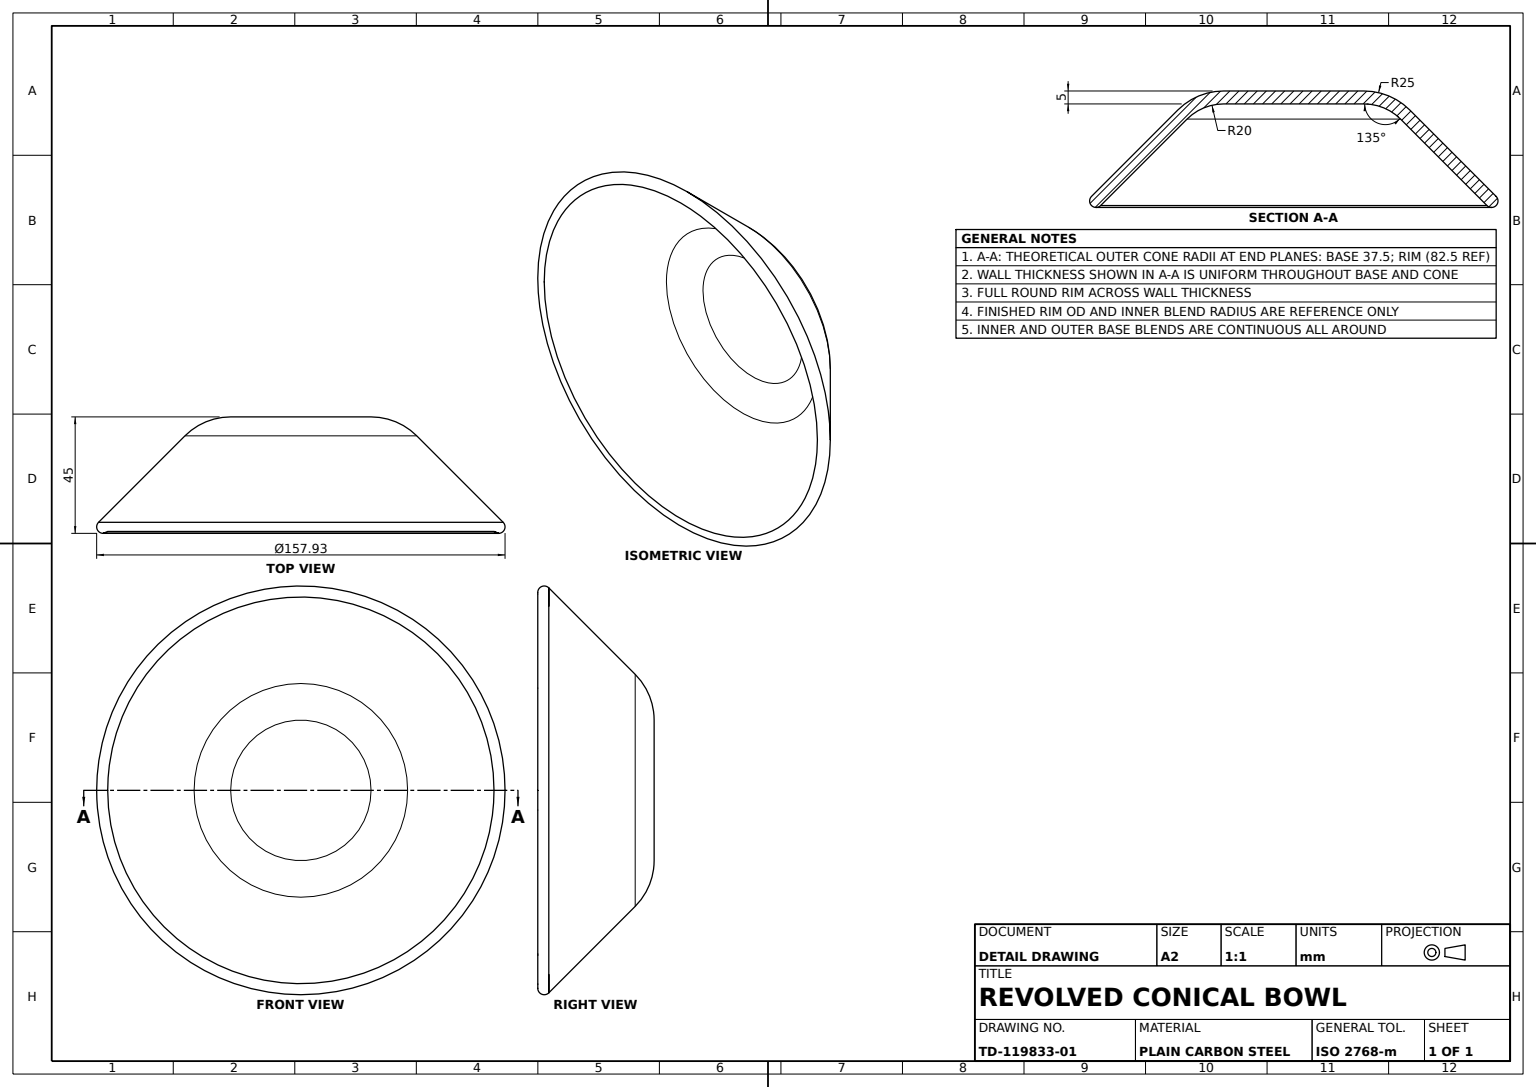
ISO-10303-21;
HEADER;
FILE_DESCRIPTION((''),'2;1');
FILE_NAME('','',(''),(''),'','','');
FILE_SCHEMA(('AUTOMOTIVE_DESIGN'));
ENDSEC;
DATA;
#1=APPLICATION_CONTEXT('');
#2=PRODUCT_CONTEXT('',#1,'mechanical');
#3=PRODUCT('','','',(#2));
#4=PRODUCT_DEFINITION_FORMATION('','',#3);
#5=PRODUCT_DEFINITION_CONTEXT('',#1,'design');
#6=PRODUCT_DEFINITION('','',#4,#5);
#7=PRODUCT_DEFINITION_SHAPE('','',#6);
#8=(LENGTH_UNIT()NAMED_UNIT(*)SI_UNIT(.MILLI.,.METRE.));
#9=(NAMED_UNIT(*)PLANE_ANGLE_UNIT()SI_UNIT($,.RADIAN.));
#10=(NAMED_UNIT(*)SI_UNIT($,.STERADIAN.)SOLID_ANGLE_UNIT());
#11=UNCERTAINTY_MEASURE_WITH_UNIT(LENGTH_MEASURE(1.E-05),#8,'distance_accuracy_value','');
#12=(GEOMETRIC_REPRESENTATION_CONTEXT(3)GLOBAL_UNCERTAINTY_ASSIGNED_CONTEXT((#11))GLOBAL_UNIT_ASSIGNED_CONTEXT((#8,#9,#10))REPRESENTATION_CONTEXT('',''));
#13=CARTESIAN_POINT('',(0.,40.732233,-78.232233));
#14=VERTEX_POINT('',#13);
#15=CARTESIAN_POINT('',(0.,44.267767,-74.696699));
#16=VERTEX_POINT('',#15);
#17=CARTESIAN_POINT('',(0.,41.910744,-79.410744));
#18=CARTESIAN_POINT('',(0.,44.267767,-80.));
#19=CARTESIAN_POINT('',(0.,46.035534,-78.232233));
#20=CARTESIAN_POINT('',(0.,45.446278,-75.87521));
#21=(BOUNDED_CURVE()B_SPLINE_CURVE(5,(#13,#17,#18,#19,#20,#15),.UNSPECIFIED.,.F.,.T.)B_SPLINE_CURVE_WITH_KNOTS((6,6),(0.,1.),.UNSPECIFIED.)CURVE()GEOMETRIC_REPRESENTATION_ITEM()RATIONAL_B_SPLINE_CURVE((1.,0.6,0.4,0.4,0.6,1.))REPRESENTATION_ITEM(''));
#22=EDGE_CURVE('',#14,#16,#21,.T.);
#23=ORIENTED_EDGE('',*,*,#22,.T.);
#24=CARTESIAN_POINT('',(0.,44.267767,74.696699));
#25=VERTEX_POINT('',#24);
#26=CARTESIAN_POINT('',(4.888888,44.267767,74.696699));
#27=CARTESIAN_POINT('',(9.777654,44.267767,74.215198));
#28=CARTESIAN_POINT('',(19.367552,44.267767,72.307648));
#29=CARTESIAN_POINT('',(24.068446,44.267767,70.881648));
#30=CARTESIAN_POINT('',(33.101932,44.267767,67.139855));
#31=CARTESIAN_POINT('',(37.434301,44.267767,64.824156));
#32=CARTESIAN_POINT('',(45.564224,44.267767,59.391915));
#33=CARTESIAN_POINT('',(49.361577,44.267767,56.275508));
#34=CARTESIAN_POINT('',(56.275508,44.267767,49.361577));
#35=CARTESIAN_POINT('',(59.391915,44.267767,45.564224));
#36=CARTESIAN_POINT('',(64.824156,44.267767,37.434301));
#37=CARTESIAN_POINT('',(67.139855,44.267767,33.101932));
#38=CARTESIAN_POINT('',(70.881648,44.267767,24.068446));
#39=CARTESIAN_POINT('',(72.307648,44.267767,19.367552));
#40=CARTESIAN_POINT('',(74.215198,44.267767,9.777654));
#41=CARTESIAN_POINT('',(74.696699,44.267767,4.888888));
#42=CARTESIAN_POINT('',(74.696699,44.267767,-4.888888));
#43=CARTESIAN_POINT('',(74.215198,44.267767,-9.777654));
#44=CARTESIAN_POINT('',(72.307648,44.267767,-19.367552));
#45=CARTESIAN_POINT('',(70.881648,44.267767,-24.068446));
#46=CARTESIAN_POINT('',(67.139855,44.267767,-33.101932));
#47=CARTESIAN_POINT('',(64.824156,44.267767,-37.434301));
#48=CARTESIAN_POINT('',(59.391915,44.267767,-45.564224));
#49=CARTESIAN_POINT('',(56.275508,44.267767,-49.361577));
#50=CARTESIAN_POINT('',(49.361577,44.267767,-56.275508));
#51=CARTESIAN_POINT('',(45.564224,44.267767,-59.391915));
#52=CARTESIAN_POINT('',(37.434301,44.267767,-64.824156));
#53=CARTESIAN_POINT('',(33.101932,44.267767,-67.139855));
#54=CARTESIAN_POINT('',(24.068446,44.267767,-70.881648));
#55=CARTESIAN_POINT('',(19.367552,44.267767,-72.307648));
#56=CARTESIAN_POINT('',(9.777654,44.267767,-74.215198));
#57=CARTESIAN_POINT('',(4.888888,44.267767,-74.696699));
#58=B_SPLINE_CURVE_WITH_KNOTS('',3,(#24,#26,#27,#28,#29,#30,#31,#32,#33,#34,#35,#36,#37,#38,#39,#40,#41,#42,#43,#44,#45,#46,#47,#48,#49,#50,#51,#52,#53,#54,#55,#56,#57,#15),.UNSPECIFIED.,.F.,.F.,(4,2,2,2,2,2,2,2,2,2,2,2,2,2,2,2,4),(0.,0.03125,0.0625,0.09375,0.125,0.15625,0.1875,0.21875,0.25,0.28125,0.3125,0.34375,0.375,0.40625,0.4375,0.46875,0.5),.UNSPECIFIED.);
#59=EDGE_CURVE('',#25,#16,#58,.T.);
#60=ORIENTED_EDGE('',*,*,#59,.F.);
#61=CARTESIAN_POINT('',(0.,40.732233,78.232233));
#62=VERTEX_POINT('',#61);
#63=CARTESIAN_POINT('',(0.,41.910744,79.410744));
#64=CARTESIAN_POINT('',(0.,44.267767,80.));
#65=CARTESIAN_POINT('',(0.,46.035534,78.232233));
#66=CARTESIAN_POINT('',(0.,45.446278,75.87521));
#67=(BOUNDED_CURVE()B_SPLINE_CURVE(5,(#61,#63,#64,#65,#66,#24),.UNSPECIFIED.,.F.,.T.)B_SPLINE_CURVE_WITH_KNOTS((6,6),(0.,1.),.UNSPECIFIED.)CURVE()GEOMETRIC_REPRESENTATION_ITEM()RATIONAL_B_SPLINE_CURVE((1.,0.6,0.4,0.4,0.6,1.))REPRESENTATION_ITEM(''));
#68=EDGE_CURVE('',#62,#25,#67,.T.);
#69=ORIENTED_EDGE('',*,*,#68,.F.);
#70=CARTESIAN_POINT('',(5.120288,40.732233,-78.232233));
#71=CARTESIAN_POINT('',(10.240449,40.732233,-77.727941));
#72=CARTESIAN_POINT('',(20.284254,40.732233,-75.730104));
#73=CARTESIAN_POINT('',(25.20765,40.732233,-74.236608));
#74=CARTESIAN_POINT('',(34.668708,40.732233,-70.31771));
#75=CARTESIAN_POINT('',(39.206136,40.732233,-67.892404));
#76=CARTESIAN_POINT('',(47.720864,40.732233,-62.203045));
#77=CARTESIAN_POINT('',(51.697952,40.732233,-58.939133));
#78=CARTESIAN_POINT('',(58.939133,40.732233,-51.697952));
#79=CARTESIAN_POINT('',(62.203045,40.732233,-47.720864));
#80=CARTESIAN_POINT('',(67.892404,40.732233,-39.206136));
#81=CARTESIAN_POINT('',(70.31771,40.732233,-34.668708));
#82=CARTESIAN_POINT('',(74.236608,40.732233,-25.20765));
#83=CARTESIAN_POINT('',(75.730104,40.732233,-20.284254));
#84=CARTESIAN_POINT('',(77.727941,40.732233,-10.240449));
#85=CARTESIAN_POINT('',(78.232233,40.732233,-5.120288));
#86=CARTESIAN_POINT('',(78.232233,40.732233,5.120288));
#87=CARTESIAN_POINT('',(77.727941,40.732233,10.240449));
#88=CARTESIAN_POINT('',(75.730104,40.732233,20.284254));
#89=CARTESIAN_POINT('',(74.236608,40.732233,25.20765));
#90=CARTESIAN_POINT('',(70.31771,40.732233,34.668708));
#91=CARTESIAN_POINT('',(67.892404,40.732233,39.206136));
#92=CARTESIAN_POINT('',(62.203045,40.732233,47.720864));
#93=CARTESIAN_POINT('',(58.939133,40.732233,51.697952));
#94=CARTESIAN_POINT('',(51.697952,40.732233,58.939133));
#95=CARTESIAN_POINT('',(47.720864,40.732233,62.203045));
#96=CARTESIAN_POINT('',(39.206136,40.732233,67.892404));
#97=CARTESIAN_POINT('',(34.668708,40.732233,70.31771));
#98=CARTESIAN_POINT('',(25.20765,40.732233,74.236608));
#99=CARTESIAN_POINT('',(20.284254,40.732233,75.730104));
#100=CARTESIAN_POINT('',(10.240449,40.732233,77.727941));
#101=CARTESIAN_POINT('',(5.120288,40.732233,78.232233));
#102=B_SPLINE_CURVE_WITH_KNOTS('',3,(#13,#70,#71,#72,#73,#74,#75,#76,#77,#78,#79,#80,#81,#82,#83,#84,#85,#86,#87,#88,#89,#90,#91,#92,#93,#94,#95,#96,#97,#98,#99,#100,#101,#61),.UNSPECIFIED.,.F.,.F.,(4,2,2,2,2,2,2,2,2,2,2,2,2,2,2,2,4),(0.5,0.53125,0.5625,0.59375,0.625,0.65625,0.6875,0.71875,0.75,0.78125,0.8125,0.84375,0.875,0.90625,0.9375,0.96875,1.),.UNSPECIFIED.);
#103=EDGE_CURVE('',#14,#62,#102,.T.);
#104=ORIENTED_EDGE('',*,*,#103,.F.);
#105=EDGE_LOOP('',(#23,#60,#69,#104));
#106=FACE_OUTER_BOUND('',#105,.T.);
#107=CARTESIAN_POINT('',(-5.116753,40.732233,78.232233));
#108=CARTESIAN_POINT('',(-10.238436,40.732233,77.728342));
#109=CARTESIAN_POINT('',(-20.286267,40.732233,75.729704));
#110=CARTESIAN_POINT('',(-25.210916,40.732233,74.235256));
#111=CARTESIAN_POINT('',(-34.665443,40.732233,70.319062));
#112=CARTESIAN_POINT('',(-39.20443,40.732233,67.893544));
#113=CARTESIAN_POINT('',(-47.72257,40.732233,62.201905));
#114=CARTESIAN_POINT('',(-51.700451,40.732233,58.936634));
#115=CARTESIAN_POINT('',(-58.936634,40.732233,51.700451));
#116=CARTESIAN_POINT('',(-62.201905,40.732233,47.72257));
#117=CARTESIAN_POINT('',(-67.893544,40.732233,39.20443));
#118=CARTESIAN_POINT('',(-70.319062,40.732233,34.665443));
#119=CARTESIAN_POINT('',(-74.235256,40.732233,25.210916));
#120=CARTESIAN_POINT('',(-75.729704,40.732233,20.286267));
#121=CARTESIAN_POINT('',(-77.728342,40.732233,10.238436));
#122=CARTESIAN_POINT('',(-78.232233,40.732233,5.116753));
#123=CARTESIAN_POINT('',(-78.232233,40.732233,-5.116753));
#124=CARTESIAN_POINT('',(-77.728342,40.732233,-10.238436));
#125=CARTESIAN_POINT('',(-75.729704,40.732233,-20.286267));
#126=CARTESIAN_POINT('',(-74.235256,40.732233,-25.210916));
#127=CARTESIAN_POINT('',(-70.319062,40.732233,-34.665443));
#128=CARTESIAN_POINT('',(-67.893544,40.732233,-39.20443));
#129=CARTESIAN_POINT('',(-62.201905,40.732233,-47.72257));
#130=CARTESIAN_POINT('',(-58.936634,40.732233,-51.700451));
#131=CARTESIAN_POINT('',(-51.700451,40.732233,-58.936634));
#132=CARTESIAN_POINT('',(-47.72257,40.732233,-62.201905));
#133=CARTESIAN_POINT('',(-39.20443,40.732233,-67.893544));
#134=CARTESIAN_POINT('',(-34.665443,40.732233,-70.319062));
#135=CARTESIAN_POINT('',(-25.210916,40.732233,-74.235256));
#136=CARTESIAN_POINT('',(-20.286267,40.732233,-75.729704));
#137=CARTESIAN_POINT('',(-10.238436,40.732233,-77.728342));
#138=CARTESIAN_POINT('',(-5.116753,40.732233,-78.232233));
#139=CARTESIAN_POINT('',(5.116753,40.732233,-78.232233));
#140=CARTESIAN_POINT('',(10.238436,40.732233,-77.728342));
#141=CARTESIAN_POINT('',(20.286267,40.732233,-75.729704));
#142=CARTESIAN_POINT('',(25.210916,40.732233,-74.235256));
#143=CARTESIAN_POINT('',(34.665443,40.732233,-70.319062));
#144=CARTESIAN_POINT('',(39.20443,40.732233,-67.893544));
#145=CARTESIAN_POINT('',(47.72257,40.732233,-62.201905));
#146=CARTESIAN_POINT('',(51.700451,40.732233,-58.936634));
#147=CARTESIAN_POINT('',(58.936634,40.732233,-51.700451));
#148=CARTESIAN_POINT('',(62.201905,40.732233,-47.72257));
#149=CARTESIAN_POINT('',(67.893544,40.732233,-39.20443));
#150=CARTESIAN_POINT('',(70.319062,40.732233,-34.665443));
#151=CARTESIAN_POINT('',(74.235256,40.732233,-25.210916));
#152=CARTESIAN_POINT('',(75.729704,40.732233,-20.286267));
#153=CARTESIAN_POINT('',(77.728342,40.732233,-10.238436));
#154=CARTESIAN_POINT('',(78.232233,40.732233,-5.116753));
#155=CARTESIAN_POINT('',(78.232233,40.732233,5.116753));
#156=CARTESIAN_POINT('',(77.728342,40.732233,10.238436));
#157=CARTESIAN_POINT('',(75.729704,40.732233,20.286267));
#158=CARTESIAN_POINT('',(74.235256,40.732233,25.210916));
#159=CARTESIAN_POINT('',(70.319062,40.732233,34.665443));
#160=CARTESIAN_POINT('',(67.893544,40.732233,39.20443));
#161=CARTESIAN_POINT('',(62.201905,40.732233,47.72257));
#162=CARTESIAN_POINT('',(58.936634,40.732233,51.700451));
#163=CARTESIAN_POINT('',(51.700451,40.732233,58.936634));
#164=CARTESIAN_POINT('',(47.72257,40.732233,62.201905));
#165=CARTESIAN_POINT('',(39.20443,40.732233,67.893544));
#166=CARTESIAN_POINT('',(34.665443,40.732233,70.319062));
#167=CARTESIAN_POINT('',(25.210916,40.732233,74.235256));
#168=CARTESIAN_POINT('',(20.286267,40.732233,75.729704));
#169=CARTESIAN_POINT('',(10.238436,40.732233,77.728342));
#170=CARTESIAN_POINT('',(5.116753,40.732233,78.232233));
#171=CARTESIAN_POINT('',(-5.194863,41.910744,79.410744));
#172=CARTESIAN_POINT('',(-10.393185,41.910744,78.89916));
#173=CARTESIAN_POINT('',(-20.591351,41.910744,76.870618));
#174=CARTESIAN_POINT('',(-25.589749,41.910744,75.353949));
#175=CARTESIAN_POINT('',(-35.188604,41.910744,71.377973));
#176=CARTESIAN_POINT('',(-39.795452,41.910744,68.916019));
#177=CARTESIAN_POINT('',(-48.44104,41.910744,63.139222));
#178=CARTESIAN_POINT('',(-52.478553,41.910744,59.825199));
#179=CARTESIAN_POINT('',(-59.825199,41.910744,52.478553));
#180=CARTESIAN_POINT('',(-63.139222,41.910744,48.44104));
#181=CARTESIAN_POINT('',(-68.916019,41.910744,39.795452));
#182=CARTESIAN_POINT('',(-71.377973,41.910744,35.188604));
#183=CARTESIAN_POINT('',(-75.353949,41.910744,25.589749));
#184=CARTESIAN_POINT('',(-76.870618,41.910744,20.591351));
#185=CARTESIAN_POINT('',(-78.89916,41.910744,10.393185));
#186=CARTESIAN_POINT('',(-79.410744,41.910744,5.194863));
#187=CARTESIAN_POINT('',(-79.410744,41.910744,-5.194863));
#188=CARTESIAN_POINT('',(-78.89916,41.910744,-10.393185));
#189=CARTESIAN_POINT('',(-76.870618,41.910744,-20.591351));
#190=CARTESIAN_POINT('',(-75.353949,41.910744,-25.589749));
#191=CARTESIAN_POINT('',(-71.377973,41.910744,-35.188604));
#192=CARTESIAN_POINT('',(-68.916019,41.910744,-39.795452));
#193=CARTESIAN_POINT('',(-63.139222,41.910744,-48.44104));
#194=CARTESIAN_POINT('',(-59.825199,41.910744,-52.478553));
#195=CARTESIAN_POINT('',(-52.478553,41.910744,-59.825199));
#196=CARTESIAN_POINT('',(-48.44104,41.910744,-63.139222));
#197=CARTESIAN_POINT('',(-39.795452,41.910744,-68.916019));
#198=CARTESIAN_POINT('',(-35.188604,41.910744,-71.377973));
#199=CARTESIAN_POINT('',(-25.589749,41.910744,-75.353949));
#200=CARTESIAN_POINT('',(-20.591351,41.910744,-76.870618));
#201=CARTESIAN_POINT('',(-10.393185,41.910744,-78.89916));
#202=CARTESIAN_POINT('',(-5.194863,41.910744,-79.410744));
#203=CARTESIAN_POINT('',(5.194863,41.910744,-79.410744));
#204=CARTESIAN_POINT('',(10.393185,41.910744,-78.89916));
#205=CARTESIAN_POINT('',(20.591351,41.910744,-76.870618));
#206=CARTESIAN_POINT('',(25.589749,41.910744,-75.353949));
#207=CARTESIAN_POINT('',(35.188604,41.910744,-71.377973));
#208=CARTESIAN_POINT('',(39.795452,41.910744,-68.916019));
#209=CARTESIAN_POINT('',(48.44104,41.910744,-63.139222));
#210=CARTESIAN_POINT('',(52.478553,41.910744,-59.825199));
#211=CARTESIAN_POINT('',(59.825199,41.910744,-52.478553));
#212=CARTESIAN_POINT('',(63.139222,41.910744,-48.44104));
#213=CARTESIAN_POINT('',(68.916019,41.910744,-39.795452));
#214=CARTESIAN_POINT('',(71.377973,41.910744,-35.188604));
#215=CARTESIAN_POINT('',(75.353949,41.910744,-25.589749));
#216=CARTESIAN_POINT('',(76.870618,41.910744,-20.591351));
#217=CARTESIAN_POINT('',(78.89916,41.910744,-10.393185));
#218=CARTESIAN_POINT('',(79.410744,41.910744,-5.194863));
#219=CARTESIAN_POINT('',(79.410744,41.910744,5.194863));
#220=CARTESIAN_POINT('',(78.89916,41.910744,10.393185));
#221=CARTESIAN_POINT('',(76.870618,41.910744,20.591351));
#222=CARTESIAN_POINT('',(75.353949,41.910744,25.589749));
#223=CARTESIAN_POINT('',(71.377973,41.910744,35.188604));
#224=CARTESIAN_POINT('',(68.916019,41.910744,39.795452));
#225=CARTESIAN_POINT('',(63.139222,41.910744,48.44104));
#226=CARTESIAN_POINT('',(59.825199,41.910744,52.478553));
#227=CARTESIAN_POINT('',(52.478553,41.910744,59.825199));
#228=CARTESIAN_POINT('',(48.44104,41.910744,63.139222));
#229=CARTESIAN_POINT('',(39.795452,41.910744,68.916019));
#230=CARTESIAN_POINT('',(35.188604,41.910744,71.377973));
#231=CARTESIAN_POINT('',(25.589749,41.910744,75.353949));
#232=CARTESIAN_POINT('',(20.591351,41.910744,76.870618));
#233=CARTESIAN_POINT('',(10.393185,41.910744,78.89916));
#234=CARTESIAN_POINT('',(5.194863,41.910744,79.410744));
#235=CARTESIAN_POINT('',(-5.233917,44.267767,80.));
#236=CARTESIAN_POINT('',(-10.470559,44.267767,79.484569));
#237=CARTESIAN_POINT('',(-20.743892,44.267767,77.441076));
#238=CARTESIAN_POINT('',(-25.779165,44.267767,75.913296));
#239=CARTESIAN_POINT('',(-35.450184,44.267767,71.907429));
#240=CARTESIAN_POINT('',(-40.090963,44.267767,69.427257));
#241=CARTESIAN_POINT('',(-48.800274,44.267767,63.607881));
#242=CARTESIAN_POINT('',(-52.867604,44.267767,60.269481));
#243=CARTESIAN_POINT('',(-60.269481,44.267767,52.867604));
#244=CARTESIAN_POINT('',(-63.607881,44.267767,48.800274));
#245=CARTESIAN_POINT('',(-69.427257,44.267767,40.090963));
#246=CARTESIAN_POINT('',(-71.907429,44.267767,35.450184));
#247=CARTESIAN_POINT('',(-75.913296,44.267767,25.779165));
#248=CARTESIAN_POINT('',(-77.441076,44.267767,20.743892));
#249=CARTESIAN_POINT('',(-79.484569,44.267767,10.470559));
#250=CARTESIAN_POINT('',(-80.,44.267767,5.233917));
#251=CARTESIAN_POINT('',(-80.,44.267767,-5.233917));
#252=CARTESIAN_POINT('',(-79.484569,44.267767,-10.470559));
#253=CARTESIAN_POINT('',(-77.441076,44.267767,-20.743892));
#254=CARTESIAN_POINT('',(-75.913296,44.267767,-25.779165));
#255=CARTESIAN_POINT('',(-71.907429,44.267767,-35.450184));
#256=CARTESIAN_POINT('',(-69.427257,44.267767,-40.090963));
#257=CARTESIAN_POINT('',(-63.607881,44.267767,-48.800274));
#258=CARTESIAN_POINT('',(-60.269481,44.267767,-52.867604));
#259=CARTESIAN_POINT('',(-52.867604,44.267767,-60.269481));
#260=CARTESIAN_POINT('',(-48.800274,44.267767,-63.607881));
#261=CARTESIAN_POINT('',(-40.090963,44.267767,-69.427257));
#262=CARTESIAN_POINT('',(-35.450184,44.267767,-71.907429));
#263=CARTESIAN_POINT('',(-25.779165,44.267767,-75.913296));
#264=CARTESIAN_POINT('',(-20.743892,44.267767,-77.441076));
#265=CARTESIAN_POINT('',(-10.470559,44.267767,-79.484569));
#266=CARTESIAN_POINT('',(-5.233917,44.267767,-80.));
#267=CARTESIAN_POINT('',(5.233917,44.267767,-80.));
#268=CARTESIAN_POINT('',(10.470559,44.267767,-79.484569));
#269=CARTESIAN_POINT('',(20.743892,44.267767,-77.441076));
#270=CARTESIAN_POINT('',(25.779165,44.267767,-75.913296));
#271=CARTESIAN_POINT('',(35.450184,44.267767,-71.907429));
#272=CARTESIAN_POINT('',(40.090963,44.267767,-69.427257));
#273=CARTESIAN_POINT('',(48.800274,44.267767,-63.607881));
#274=CARTESIAN_POINT('',(52.867604,44.267767,-60.269481));
#275=CARTESIAN_POINT('',(60.269481,44.267767,-52.867604));
#276=CARTESIAN_POINT('',(63.607881,44.267767,-48.800274));
#277=CARTESIAN_POINT('',(69.427257,44.267767,-40.090963));
#278=CARTESIAN_POINT('',(71.907429,44.267767,-35.450184));
#279=CARTESIAN_POINT('',(75.913296,44.267767,-25.779165));
#280=CARTESIAN_POINT('',(77.441076,44.267767,-20.743892));
#281=CARTESIAN_POINT('',(79.484569,44.267767,-10.470559));
#282=CARTESIAN_POINT('',(80.,44.267767,-5.233917));
#283=CARTESIAN_POINT('',(80.,44.267767,5.233917));
#284=CARTESIAN_POINT('',(79.484569,44.267767,10.470559));
#285=CARTESIAN_POINT('',(77.441076,44.267767,20.743892));
#286=CARTESIAN_POINT('',(75.913296,44.267767,25.779165));
#287=CARTESIAN_POINT('',(71.907429,44.267767,35.450184));
#288=CARTESIAN_POINT('',(69.427257,44.267767,40.090963));
#289=CARTESIAN_POINT('',(63.607881,44.267767,48.800274));
#290=CARTESIAN_POINT('',(60.269481,44.267767,52.867604));
#291=CARTESIAN_POINT('',(52.867604,44.267767,60.269481));
#292=CARTESIAN_POINT('',(48.800274,44.267767,63.607881));
#293=CARTESIAN_POINT('',(40.090963,44.267767,69.427257));
#294=CARTESIAN_POINT('',(35.450184,44.267767,71.907429));
#295=CARTESIAN_POINT('',(25.779165,44.267767,75.913296));
#296=CARTESIAN_POINT('',(20.743892,44.267767,77.441076));
#297=CARTESIAN_POINT('',(10.470559,44.267767,79.484569));
#298=CARTESIAN_POINT('',(5.233917,44.267767,80.));
#299=CARTESIAN_POINT('',(-5.116753,46.035534,78.232233));
#300=CARTESIAN_POINT('',(-10.238436,46.035534,77.728342));
#301=CARTESIAN_POINT('',(-20.286267,46.035534,75.729704));
#302=CARTESIAN_POINT('',(-25.210916,46.035534,74.235256));
#303=CARTESIAN_POINT('',(-34.665443,46.035534,70.319062));
#304=CARTESIAN_POINT('',(-39.20443,46.035534,67.893544));
#305=CARTESIAN_POINT('',(-47.72257,46.035534,62.201905));
#306=CARTESIAN_POINT('',(-51.700451,46.035534,58.936634));
#307=CARTESIAN_POINT('',(-58.936634,46.035534,51.700451));
#308=CARTESIAN_POINT('',(-62.201905,46.035534,47.72257));
#309=CARTESIAN_POINT('',(-67.893544,46.035534,39.20443));
#310=CARTESIAN_POINT('',(-70.319062,46.035534,34.665443));
#311=CARTESIAN_POINT('',(-74.235256,46.035534,25.210916));
#312=CARTESIAN_POINT('',(-75.729704,46.035534,20.286267));
#313=CARTESIAN_POINT('',(-77.728342,46.035534,10.238436));
#314=CARTESIAN_POINT('',(-78.232233,46.035534,5.116753));
#315=CARTESIAN_POINT('',(-78.232233,46.035534,-5.116753));
#316=CARTESIAN_POINT('',(-77.728342,46.035534,-10.238436));
#317=CARTESIAN_POINT('',(-75.729704,46.035534,-20.286267));
#318=CARTESIAN_POINT('',(-74.235256,46.035534,-25.210916));
#319=CARTESIAN_POINT('',(-70.319062,46.035534,-34.665443));
#320=CARTESIAN_POINT('',(-67.893544,46.035534,-39.20443));
#321=CARTESIAN_POINT('',(-62.201905,46.035534,-47.72257));
#322=CARTESIAN_POINT('',(-58.936634,46.035534,-51.700451));
#323=CARTESIAN_POINT('',(-51.700451,46.035534,-58.936634));
#324=CARTESIAN_POINT('',(-47.72257,46.035534,-62.201905));
#325=CARTESIAN_POINT('',(-39.20443,46.035534,-67.893544));
#326=CARTESIAN_POINT('',(-34.665443,46.035534,-70.319062));
#327=CARTESIAN_POINT('',(-25.210916,46.035534,-74.235256));
#328=CARTESIAN_POINT('',(-20.286267,46.035534,-75.729704));
#329=CARTESIAN_POINT('',(-10.238436,46.035534,-77.728342));
#330=CARTESIAN_POINT('',(-5.116753,46.035534,-78.232233));
#331=CARTESIAN_POINT('',(5.116753,46.035534,-78.232233));
#332=CARTESIAN_POINT('',(10.238436,46.035534,-77.728342));
#333=CARTESIAN_POINT('',(20.286267,46.035534,-75.729704));
#334=CARTESIAN_POINT('',(25.210916,46.035534,-74.235256));
#335=CARTESIAN_POINT('',(34.665443,46.035534,-70.319062));
#336=CARTESIAN_POINT('',(39.20443,46.035534,-67.893544));
#337=CARTESIAN_POINT('',(47.72257,46.035534,-62.201905));
#338=CARTESIAN_POINT('',(51.700451,46.035534,-58.936634));
#339=CARTESIAN_POINT('',(58.936634,46.035534,-51.700451));
#340=CARTESIAN_POINT('',(62.201905,46.035534,-47.72257));
#341=CARTESIAN_POINT('',(67.893544,46.035534,-39.20443));
#342=CARTESIAN_POINT('',(70.319062,46.035534,-34.665443));
#343=CARTESIAN_POINT('',(74.235256,46.035534,-25.210916));
#344=CARTESIAN_POINT('',(75.729704,46.035534,-20.286267));
#345=CARTESIAN_POINT('',(77.728342,46.035534,-10.238436));
#346=CARTESIAN_POINT('',(78.232233,46.035534,-5.116753));
#347=CARTESIAN_POINT('',(78.232233,46.035534,5.116753));
#348=CARTESIAN_POINT('',(77.728342,46.035534,10.238436));
#349=CARTESIAN_POINT('',(75.729704,46.035534,20.286267));
#350=CARTESIAN_POINT('',(74.235256,46.035534,25.210916));
#351=CARTESIAN_POINT('',(70.319062,46.035534,34.665443));
#352=CARTESIAN_POINT('',(67.893544,46.035534,39.20443));
#353=CARTESIAN_POINT('',(62.201905,46.035534,47.72257));
#354=CARTESIAN_POINT('',(58.936634,46.035534,51.700451));
#355=CARTESIAN_POINT('',(51.700451,46.035534,58.936634));
#356=CARTESIAN_POINT('',(47.72257,46.035534,62.201905));
#357=CARTESIAN_POINT('',(39.20443,46.035534,67.893544));
#358=CARTESIAN_POINT('',(34.665443,46.035534,70.319062));
#359=CARTESIAN_POINT('',(25.210916,46.035534,74.235256));
#360=CARTESIAN_POINT('',(20.286267,46.035534,75.729704));
#361=CARTESIAN_POINT('',(10.238436,46.035534,77.728342));
#362=CARTESIAN_POINT('',(5.116753,46.035534,78.232233));
#363=CARTESIAN_POINT('',(-4.960535,45.446278,75.87521));
#364=CARTESIAN_POINT('',(-9.928937,45.446278,75.386705));
#365=CARTESIAN_POINT('',(-19.676101,45.446278,73.447874));
#366=CARTESIAN_POINT('',(-24.453249,45.446278,71.997868));
#367=CARTESIAN_POINT('',(-33.619123,45.446278,68.201239));
#368=CARTESIAN_POINT('',(-38.022385,45.446278,65.848594));
#369=CARTESIAN_POINT('',(-46.285632,45.446278,60.327269));
#370=CARTESIAN_POINT('',(-50.144248,45.446278,57.159504));
#371=CARTESIAN_POINT('',(-57.159504,45.446278,50.144248));
#372=CARTESIAN_POINT('',(-60.327269,45.446278,46.285632));
#373=CARTESIAN_POINT('',(-65.848594,45.446278,38.022385));
#374=CARTESIAN_POINT('',(-68.201239,45.446278,33.619123));
#375=CARTESIAN_POINT('',(-71.997868,45.446278,24.453249));
#376=CARTESIAN_POINT('',(-73.447874,45.446278,19.676101));
#377=CARTESIAN_POINT('',(-75.386705,45.446278,9.928937));
#378=CARTESIAN_POINT('',(-75.87521,45.446278,4.960535));
#379=CARTESIAN_POINT('',(-75.87521,45.446278,-4.960535));
#380=CARTESIAN_POINT('',(-75.386705,45.446278,-9.928937));
#381=CARTESIAN_POINT('',(-73.447874,45.446278,-19.676101));
#382=CARTESIAN_POINT('',(-71.997868,45.446278,-24.453249));
#383=CARTESIAN_POINT('',(-68.201239,45.446278,-33.619123));
#384=CARTESIAN_POINT('',(-65.848594,45.446278,-38.022385));
#385=CARTESIAN_POINT('',(-60.327269,45.446278,-46.285632));
#386=CARTESIAN_POINT('',(-57.159504,45.446278,-50.144248));
#387=CARTESIAN_POINT('',(-50.144248,45.446278,-57.159504));
#388=CARTESIAN_POINT('',(-46.285632,45.446278,-60.327269));
#389=CARTESIAN_POINT('',(-38.022385,45.446278,-65.848594));
#390=CARTESIAN_POINT('',(-33.619123,45.446278,-68.201239));
#391=CARTESIAN_POINT('',(-24.453249,45.446278,-71.997868));
#392=CARTESIAN_POINT('',(-19.676101,45.446278,-73.447874));
#393=CARTESIAN_POINT('',(-9.928937,45.446278,-75.386705));
#394=CARTESIAN_POINT('',(-4.960535,45.446278,-75.87521));
#395=CARTESIAN_POINT('',(4.960535,45.446278,-75.87521));
#396=CARTESIAN_POINT('',(9.928937,45.446278,-75.386705));
#397=CARTESIAN_POINT('',(19.676101,45.446278,-73.447874));
#398=CARTESIAN_POINT('',(24.453249,45.446278,-71.997868));
#399=CARTESIAN_POINT('',(33.619123,45.446278,-68.201239));
#400=CARTESIAN_POINT('',(38.022385,45.446278,-65.848594));
#401=CARTESIAN_POINT('',(46.285632,45.446278,-60.327269));
#402=CARTESIAN_POINT('',(50.144248,45.446278,-57.159504));
#403=CARTESIAN_POINT('',(57.159504,45.446278,-50.144248));
#404=CARTESIAN_POINT('',(60.327269,45.446278,-46.285632));
#405=CARTESIAN_POINT('',(65.848594,45.446278,-38.022385));
#406=CARTESIAN_POINT('',(68.201239,45.446278,-33.619123));
#407=CARTESIAN_POINT('',(71.997868,45.446278,-24.453249));
#408=CARTESIAN_POINT('',(73.447874,45.446278,-19.676101));
#409=CARTESIAN_POINT('',(75.386705,45.446278,-9.928937));
#410=CARTESIAN_POINT('',(75.87521,45.446278,-4.960535));
#411=CARTESIAN_POINT('',(75.87521,45.446278,4.960535));
#412=CARTESIAN_POINT('',(75.386705,45.446278,9.928937));
#413=CARTESIAN_POINT('',(73.447874,45.446278,19.676101));
#414=CARTESIAN_POINT('',(71.997868,45.446278,24.453249));
#415=CARTESIAN_POINT('',(68.201239,45.446278,33.619123));
#416=CARTESIAN_POINT('',(65.848594,45.446278,38.022385));
#417=CARTESIAN_POINT('',(60.327269,45.446278,46.285632));
#418=CARTESIAN_POINT('',(57.159504,45.446278,50.144248));
#419=CARTESIAN_POINT('',(50.144248,45.446278,57.159504));
#420=CARTESIAN_POINT('',(46.285632,45.446278,60.327269));
#421=CARTESIAN_POINT('',(38.022385,45.446278,65.848594));
#422=CARTESIAN_POINT('',(33.619123,45.446278,68.201239));
#423=CARTESIAN_POINT('',(24.453249,45.446278,71.997868));
#424=CARTESIAN_POINT('',(19.676101,45.446278,73.447874));
#425=CARTESIAN_POINT('',(9.928937,45.446278,75.386705));
#426=CARTESIAN_POINT('',(4.960535,45.446278,75.87521));
#427=CARTESIAN_POINT('',(-4.882425,44.267767,74.696699));
#428=CARTESIAN_POINT('',(-9.774188,44.267767,74.215887));
#429=CARTESIAN_POINT('',(-19.371018,44.267767,72.306959));
#430=CARTESIAN_POINT('',(-24.074416,44.267767,70.879175));
#431=CARTESIAN_POINT('',(-33.095962,44.267767,67.142328));
#432=CARTESIAN_POINT('',(-37.431363,44.267767,64.826119));
#433=CARTESIAN_POINT('',(-45.567162,44.267767,59.389952));
#434=CARTESIAN_POINT('',(-49.366146,44.267767,56.270939));
#435=CARTESIAN_POINT('',(-56.270939,44.267767,49.366146));
#436=CARTESIAN_POINT('',(-59.389952,44.267767,45.567162));
#437=CARTESIAN_POINT('',(-64.826119,44.267767,37.431363));
#438=CARTESIAN_POINT('',(-67.142328,44.267767,33.095962));
#439=CARTESIAN_POINT('',(-70.879175,44.267767,24.074416));
#440=CARTESIAN_POINT('',(-72.306959,44.267767,19.371018));
#441=CARTESIAN_POINT('',(-74.215887,44.267767,9.774188));
#442=CARTESIAN_POINT('',(-74.696699,44.267767,4.882425));
#443=CARTESIAN_POINT('',(-74.696699,44.267767,-4.882425));
#444=CARTESIAN_POINT('',(-74.215887,44.267767,-9.774188));
#445=CARTESIAN_POINT('',(-72.306959,44.267767,-19.371018));
#446=CARTESIAN_POINT('',(-70.879175,44.267767,-24.074416));
#447=CARTESIAN_POINT('',(-67.142328,44.267767,-33.095962));
#448=CARTESIAN_POINT('',(-64.826119,44.267767,-37.431363));
#449=CARTESIAN_POINT('',(-59.389952,44.267767,-45.567162));
#450=CARTESIAN_POINT('',(-56.270939,44.267767,-49.366146));
#451=CARTESIAN_POINT('',(-49.366146,44.267767,-56.270939));
#452=CARTESIAN_POINT('',(-45.567162,44.267767,-59.389952));
#453=CARTESIAN_POINT('',(-37.431363,44.267767,-64.826119));
#454=CARTESIAN_POINT('',(-33.095962,44.267767,-67.142328));
#455=CARTESIAN_POINT('',(-24.074416,44.267767,-70.879175));
#456=CARTESIAN_POINT('',(-19.371018,44.267767,-72.306959));
#457=CARTESIAN_POINT('',(-9.774188,44.267767,-74.215887));
#458=CARTESIAN_POINT('',(-4.882425,44.267767,-74.696699));
#459=CARTESIAN_POINT('',(4.882425,44.267767,-74.696699));
#460=CARTESIAN_POINT('',(9.774188,44.267767,-74.215887));
#461=CARTESIAN_POINT('',(19.371018,44.267767,-72.306959));
#462=CARTESIAN_POINT('',(24.074416,44.267767,-70.879175));
#463=CARTESIAN_POINT('',(33.095962,44.267767,-67.142328));
#464=CARTESIAN_POINT('',(37.431363,44.267767,-64.826119));
#465=CARTESIAN_POINT('',(45.567162,44.267767,-59.389952));
#466=CARTESIAN_POINT('',(49.366146,44.267767,-56.270939));
#467=CARTESIAN_POINT('',(56.270939,44.267767,-49.366146));
#468=CARTESIAN_POINT('',(59.389952,44.267767,-45.567162));
#469=CARTESIAN_POINT('',(64.826119,44.267767,-37.431363));
#470=CARTESIAN_POINT('',(67.142328,44.267767,-33.095962));
#471=CARTESIAN_POINT('',(70.879175,44.267767,-24.074416));
#472=CARTESIAN_POINT('',(72.306959,44.267767,-19.371018));
#473=CARTESIAN_POINT('',(74.215887,44.267767,-9.774188));
#474=CARTESIAN_POINT('',(74.696699,44.267767,-4.882425));
#475=CARTESIAN_POINT('',(74.696699,44.267767,4.882425));
#476=CARTESIAN_POINT('',(74.215887,44.267767,9.774188));
#477=CARTESIAN_POINT('',(72.306959,44.267767,19.371018));
#478=CARTESIAN_POINT('',(70.879175,44.267767,24.074416));
#479=CARTESIAN_POINT('',(67.142328,44.267767,33.095962));
#480=CARTESIAN_POINT('',(64.826119,44.267767,37.431363));
#481=CARTESIAN_POINT('',(59.389952,44.267767,45.567162));
#482=CARTESIAN_POINT('',(56.270939,44.267767,49.366146));
#483=CARTESIAN_POINT('',(49.366146,44.267767,56.270939));
#484=CARTESIAN_POINT('',(45.567162,44.267767,59.389952));
#485=CARTESIAN_POINT('',(37.431363,44.267767,64.826119));
#486=CARTESIAN_POINT('',(33.095962,44.267767,67.142328));
#487=CARTESIAN_POINT('',(24.074416,44.267767,70.879175));
#488=CARTESIAN_POINT('',(19.371018,44.267767,72.306959));
#489=CARTESIAN_POINT('',(9.774188,44.267767,74.215887));
#490=CARTESIAN_POINT('',(4.882425,44.267767,74.696699));
#491=(BOUNDED_SURFACE()B_SPLINE_SURFACE(5,3,((#61,#107,#108,#109,#110,#111,#112,#113,#114,#115,#116,#117,#118,#119,#120,#121,#122,#123,#124,#125,#126,#127,#128,#129,#130,#131,#132,#133,#134,#135,#136,#137,#138,#139,#140,#141,#142,#143,#144,#145,#146,#147,#148,#149,#150,#151,#152,#153,#154,#155,#156,#157,#158,#159,#160,#161,#162,#163,#164,#165,#166,#167,#168,#169,#170,#61),(#63,#171,#172,#173,#174,#175,#176,#177,#178,#179,#180,#181,#182,#183,#184,#185,#186,#187,#188,#189,#190,#191,#192,#193,#194,#195,#196,#197,#198,#199,#200,#201,#202,#203,#204,#205,#206,#207,#208,#209,#210,#211,#212,#213,#214,#215,#216,#217,#218,#219,#220,#221,#222,#223,#224,#225,#226,#227,#228,#229,#230,#231,#232,#233,#234,#63),(#64,#235,#236,#237,#238,#239,#240,#241,#242,#243,#244,#245,#246,#247,#248,#249,#250,#251,#252,#253,#254,#255,#256,#257,#258,#259,#260,#261,#262,#263,#264,#265,#266,#267,#268,#269,#270,#271,#272,#273,#274,#275,#276,#277,#278,#279,#280,#281,#282,#283,#284,#285,#286,#287,#288,#289,#290,#291,#292,#293,#294,#295,#296,#297,#298,#64),(#65,#299,#300,#301,#302,#303,#304,#305,#306,#307,#308,#309,#310,#311,#312,#313,#314,#315,#316,#317,#318,#319,#320,#321,#322,#323,#324,#325,#326,#327,#328,#329,#330,#331,#332,#333,#334,#335,#336,#337,#338,#339,#340,#341,#342,#343,#344,#345,#346,#347,#348,#349,#350,#351,#352,#353,#354,#355,#356,#357,#358,#359,#360,#361,#362,#65),(#66,#363,#364,#365,#366,#367,#368,#369,#370,#371,#372,#373,#374,#375,#376,#377,#378,#379,#380,#381,#382,#383,#384,#385,#386,#387,#388,#389,#390,#391,#392,#393,#394,#395,#396,#397,#398,#399,#400,#401,#402,#403,#404,#405,#406,#407,#408,#409,#410,#411,#412,#413,#414,#415,#416,#417,#418,#419,#420,#421,#422,#423,#424,#425,#426,#66),(#24,#427,#428,#429,#430,#431,#432,#433,#434,#435,#436,#437,#438,#439,#440,#441,#442,#443,#444,#445,#446,#447,#448,#449,#450,#451,#452,#453,#454,#455,#456,#457,#458,#459,#460,#461,#462,#463,#464,#465,#466,#467,#468,#469,#470,#471,#472,#473,#474,#475,#476,#477,#478,#479,#480,#481,#482,#483,#484,#485,#486,#487,#488,#489,#490,#24)),.UNSPECIFIED.,.F.,.T.,.F.)B_SPLINE_SURFACE_WITH_KNOTS((6,6),(4,2,2,2,2,2,2,2,2,2,2,2,2,2,2,2,2,2,2,2,2,2,2,2,2,2,2,2,2,2,2,2,4),(0.,1.),(0.5,0.53125,0.5625,0.59375,0.625,0.65625,0.6875,0.71875,0.75,0.78125,0.8125,0.84375,0.875,0.90625,0.9375,0.96875,1.,1.03125,1.0625,1.09375,1.125,1.15625,1.1875,1.21875,1.25,1.28125,1.3125,1.34375,1.375,1.40625,1.4375,1.46875,1.5),.UNSPECIFIED.)GEOMETRIC_REPRESENTATION_ITEM()RATIONAL_B_SPLINE_SURFACE(((1.,1.,1.,1.,1.,1.,1.,1.,1.,1.,1.,1.,1.,1.,1.,1.,1.,1.,1.,1.,1.,1.,1.,1.,1.,1.,1.,1.,1.,1.,1.,1.,1.,1.,1.,1.,1.,1.,1.,1.,1.,1.,1.,1.,1.,1.,1.,1.,1.,1.,1.,1.,1.,1.,1.,1.,1.,1.,1.,1.,1.,1.,1.,1.,1.,1.),(0.6,0.6,0.6,0.6,0.6,0.6,0.6,0.6,0.6,0.6,0.6,0.6,0.6,0.6,0.6,0.6,0.6,0.6,0.6,0.6,0.6,0.6,0.6,0.6,0.6,0.6,0.6,0.6,0.6,0.6,0.6,0.6,0.6,0.6,0.6,0.6,0.6,0.6,0.6,0.6,0.6,0.6,0.6,0.6,0.6,0.6,0.6,0.6,0.6,0.6,0.6,0.6,0.6,0.6,0.6,0.6,0.6,0.6,0.6,0.6,0.6,0.6,0.6,0.6,0.6,0.6),(0.4,0.4,0.4,0.4,0.4,0.4,0.4,0.4,0.4,0.4,0.4,0.4,0.4,0.4,0.4,0.4,0.4,0.4,0.4,0.4,0.4,0.4,0.4,0.4,0.4,0.4,0.4,0.4,0.4,0.4,0.4,0.4,0.4,0.4,0.4,0.4,0.4,0.4,0.4,0.4,0.4,0.4,0.4,0.4,0.4,0.4,0.4,0.4,0.4,0.4,0.4,0.4,0.4,0.4,0.4,0.4,0.4,0.4,0.4,0.4,0.4,0.4,0.4,0.4,0.4,0.4),(0.4,0.4,0.4,0.4,0.4,0.4,0.4,0.4,0.4,0.4,0.4,0.4,0.4,0.4,0.4,0.4,0.4,0.4,0.4,0.4,0.4,0.4,0.4,0.4,0.4,0.4,0.4,0.4,0.4,0.4,0.4,0.4,0.4,0.4,0.4,0.4,0.4,0.4,0.4,0.4,0.4,0.4,0.4,0.4,0.4,0.4,0.4,0.4,0.4,0.4,0.4,0.4,0.4,0.4,0.4,0.4,0.4,0.4,0.4,0.4,0.4,0.4,0.4,0.4,0.4,0.4),(0.6,0.6,0.6,0.6,0.6,0.6,0.6,0.6,0.6,0.6,0.6,0.6,0.6,0.6,0.6,0.6,0.6,0.6,0.6,0.6,0.6,0.6,0.6,0.6,0.6,0.6,0.6,0.6,0.6,0.6,0.6,0.6,0.6,0.6,0.6,0.6,0.6,0.6,0.6,0.6,0.6,0.6,0.6,0.6,0.6,0.6,0.6,0.6,0.6,0.6,0.6,0.6,0.6,0.6,0.6,0.6,0.6,0.6,0.6,0.6,0.6,0.6,0.6,0.6,0.6,0.6),(1.,1.,1.,1.,1.,1.,1.,1.,1.,1.,1.,1.,1.,1.,1.,1.,1.,1.,1.,1.,1.,1.,1.,1.,1.,1.,1.,1.,1.,1.,1.,1.,1.,1.,1.,1.,1.,1.,1.,1.,1.,1.,1.,1.,1.,1.,1.,1.,1.,1.,1.,1.,1.,1.,1.,1.,1.,1.,1.,1.,1.,1.,1.,1.,1.,1.)))REPRESENTATION_ITEM('')SURFACE());
#492=ADVANCED_FACE('',(#106),#491,.T.);
#493=CARTESIAN_POINT('',(0.,0.,-27.144661));
#494=VERTEX_POINT('',#493);
#495=CARTESIAN_POINT('',(0.,0.,27.144661));
#496=VERTEX_POINT('',#495);
#497=CARTESIAN_POINT('',(0.,0.,0.));
#498=DIRECTION('',(0.,-1.,0.));
#499=DIRECTION('',(0.,0.,1.));
#500=AXIS2_PLACEMENT_3D('',#497,#498,#499);
#501=CIRCLE('',#500,27.144661);
#502=EDGE_CURVE('',#494,#496,#501,.T.);
#503=ORIENTED_EDGE('',*,*,#502,.T.);
#504=EDGE_CURVE('',#496,#494,#501,.T.);
#505=ORIENTED_EDGE('',*,*,#504,.T.);
#506=EDGE_LOOP('',(#503,#505));
#507=FACE_OUTER_BOUND('',#506,.T.);
#508=DIRECTION('',(0.,1.,0.));
#509=AXIS2_PLACEMENT_3D('',#497,#508,#499);
#510=PLANE('',#509);
#511=ADVANCED_FACE('',(#507),#510,.F.);
#512=CARTESIAN_POINT('',(0.,5.,27.144661));
#513=VERTEX_POINT('',#512);
#514=CARTESIAN_POINT('',(0.,10.857864,41.286797));
#515=VERTEX_POINT('',#514);
#516=CARTESIAN_POINT('',(0.,25.,27.144661));
#517=DIRECTION('',(-1.,0.,0.));
#518=AXIS2_PLACEMENT_3D('',#516,#517,#499);
#519=CIRCLE('',#518,20.);
#520=EDGE_CURVE('',#513,#515,#519,.T.);
#521=ORIENTED_EDGE('',*,*,#520,.F.);
#522=CARTESIAN_POINT('',(0.,5.,-27.144661));
#523=VERTEX_POINT('',#522);
#524=CARTESIAN_POINT('',(0.,5.,0.));
#525=AXIS2_PLACEMENT_3D('',#524,#508,#499);
#526=CIRCLE('',#525,27.144661);
#527=EDGE_CURVE('',#523,#513,#526,.T.);
#528=ORIENTED_EDGE('',*,*,#527,.F.);
#529=CARTESIAN_POINT('',(0.,10.857864,-41.286797));
#530=VERTEX_POINT('',#529);
#531=CARTESIAN_POINT('',(0.,25.,-27.144661));
#532=DIRECTION('',(1.,0.,0.));
#533=DIRECTION('',(0.,0.,-1.));
#534=AXIS2_PLACEMENT_3D('',#531,#532,#533);
#535=CIRCLE('',#534,20.);
#536=EDGE_CURVE('',#523,#530,#535,.T.);
#537=ORIENTED_EDGE('',*,*,#536,.T.);
#538=CARTESIAN_POINT('',(0.,10.857864,0.));
#539=AXIS2_PLACEMENT_3D('',#538,#508,#499);
#540=CIRCLE('',#539,41.286797);
#541=EDGE_CURVE('',#530,#515,#540,.T.);
#542=ORIENTED_EDGE('',*,*,#541,.T.);
#543=EDGE_LOOP('',(#521,#528,#537,#542));
#544=FACE_OUTER_BOUND('',#543,.T.);
#545=CARTESIAN_POINT('',(0.,25.,0.));
#546=AXIS2_PLACEMENT_3D('',#545,#508,#499);
#547=TOROIDAL_SURFACE('',#546,27.144661,20.);
#548=ADVANCED_FACE('',(#544),#547,.F.);
#549=CARTESIAN_POINT('',(0.,7.32233,-44.82233));
#550=VERTEX_POINT('',#549);
#551=CARTESIAN_POINT('',(0.,7.32233,44.82233));
#552=VERTEX_POINT('',#551);
#553=CARTESIAN_POINT('',(0.,7.32233,0.));
#554=AXIS2_PLACEMENT_3D('',#553,#508,#533);
#555=CIRCLE('',#554,44.82233);
#556=EDGE_CURVE('',#550,#552,#555,.T.);
#557=ORIENTED_EDGE('',*,*,#556,.T.);
#558=CARTESIAN_POINT('',(0.,45.,82.5));
#559=DIRECTION('',(0.,0.707106781,0.707106781));
#560=VECTOR('',#559,1000.);
#561=LINE('',#558,#560);
#562=EDGE_CURVE('',#552,#62,#561,.T.);
#563=ORIENTED_EDGE('',*,*,#562,.T.);
#564=CARTESIAN_POINT('',(-5.120288,40.732233,78.232233));
#565=CARTESIAN_POINT('',(-10.240449,40.732233,77.727941));
#566=CARTESIAN_POINT('',(-20.284254,40.732233,75.730104));
#567=CARTESIAN_POINT('',(-25.20765,40.732233,74.236608));
#568=CARTESIAN_POINT('',(-34.668708,40.732233,70.31771));
#569=CARTESIAN_POINT('',(-39.206136,40.732233,67.892404));
#570=CARTESIAN_POINT('',(-47.720864,40.732233,62.203045));
#571=CARTESIAN_POINT('',(-51.697952,40.732233,58.939133));
#572=CARTESIAN_POINT('',(-58.939133,40.732233,51.697952));
#573=CARTESIAN_POINT('',(-62.203045,40.732233,47.720864));
#574=CARTESIAN_POINT('',(-67.892404,40.732233,39.206136));
#575=CARTESIAN_POINT('',(-70.31771,40.732233,34.668708));
#576=CARTESIAN_POINT('',(-74.236608,40.732233,25.20765));
#577=CARTESIAN_POINT('',(-75.730104,40.732233,20.284254));
#578=CARTESIAN_POINT('',(-77.727941,40.732233,10.240449));
#579=CARTESIAN_POINT('',(-78.232233,40.732233,5.120288));
#580=CARTESIAN_POINT('',(-78.232233,40.732233,-5.120288));
#581=CARTESIAN_POINT('',(-77.727941,40.732233,-10.240449));
#582=CARTESIAN_POINT('',(-75.730104,40.732233,-20.284254));
#583=CARTESIAN_POINT('',(-74.236608,40.732233,-25.20765));
#584=CARTESIAN_POINT('',(-70.31771,40.732233,-34.668708));
#585=CARTESIAN_POINT('',(-67.892404,40.732233,-39.206136));
#586=CARTESIAN_POINT('',(-62.203045,40.732233,-47.720864));
#587=CARTESIAN_POINT('',(-58.939133,40.732233,-51.697952));
#588=CARTESIAN_POINT('',(-51.697952,40.732233,-58.939133));
#589=CARTESIAN_POINT('',(-47.720864,40.732233,-62.203045));
#590=CARTESIAN_POINT('',(-39.206136,40.732233,-67.892404));
#591=CARTESIAN_POINT('',(-34.668708,40.732233,-70.31771));
#592=CARTESIAN_POINT('',(-25.20765,40.732233,-74.236608));
#593=CARTESIAN_POINT('',(-20.284254,40.732233,-75.730104));
#594=CARTESIAN_POINT('',(-10.240449,40.732233,-77.727941));
#595=CARTESIAN_POINT('',(-5.120288,40.732233,-78.232233));
#596=B_SPLINE_CURVE_WITH_KNOTS('',3,(#61,#564,#565,#566,#567,#568,#569,#570,#571,#572,#573,#574,#575,#576,#577,#578,#579,#580,#581,#582,#583,#584,#585,#586,#587,#588,#589,#590,#591,#592,#593,#594,#595,#13),.UNSPECIFIED.,.F.,.F.,(4,2,2,2,2,2,2,2,2,2,2,2,2,2,2,2,4),(0.,0.03125,0.0625,0.09375,0.125,0.15625,0.1875,0.21875,0.25,0.28125,0.3125,0.34375,0.375,0.40625,0.4375,0.46875,0.5),.UNSPECIFIED.);
#597=EDGE_CURVE('',#62,#14,#596,.T.);
#598=ORIENTED_EDGE('',*,*,#597,.T.);
#599=CARTESIAN_POINT('',(0.,45.,-82.5));
#600=DIRECTION('',(0.,0.707106781,-0.707106781));
#601=VECTOR('',#600,1000.);
#602=LINE('',#599,#601);
#603=EDGE_CURVE('',#550,#14,#602,.T.);
#604=ORIENTED_EDGE('',*,*,#603,.F.);
#605=EDGE_LOOP('',(#557,#563,#598,#604));
#606=FACE_OUTER_BOUND('',#605,.T.);
#607=CARTESIAN_POINT('',(0.,45.,0.));
#608=AXIS2_PLACEMENT_3D('',#607,#508,#499);
#609=CONICAL_SURFACE('',#608,82.5,0.785398163);
#610=ADVANCED_FACE('',(#606),#609,.T.);
#611=CARTESIAN_POINT('',(0.,48.535534,-78.964466));
#612=LINE('',#611,#601);
#613=EDGE_CURVE('',#530,#16,#612,.T.);
#614=ORIENTED_EDGE('',*,*,#613,.T.);
#615=CARTESIAN_POINT('',(-4.888888,44.267767,-74.696699));
#616=CARTESIAN_POINT('',(-9.777654,44.267767,-74.215198));
#617=CARTESIAN_POINT('',(-19.367552,44.267767,-72.307648));
#618=CARTESIAN_POINT('',(-24.068446,44.267767,-70.881648));
#619=CARTESIAN_POINT('',(-33.101932,44.267767,-67.139855));
#620=CARTESIAN_POINT('',(-37.434301,44.267767,-64.824156));
#621=CARTESIAN_POINT('',(-45.564224,44.267767,-59.391915));
#622=CARTESIAN_POINT('',(-49.361577,44.267767,-56.275508));
#623=CARTESIAN_POINT('',(-56.275508,44.267767,-49.361577));
#624=CARTESIAN_POINT('',(-59.391915,44.267767,-45.564224));
#625=CARTESIAN_POINT('',(-64.824156,44.267767,-37.434301));
#626=CARTESIAN_POINT('',(-67.139855,44.267767,-33.101932));
#627=CARTESIAN_POINT('',(-70.881648,44.267767,-24.068446));
#628=CARTESIAN_POINT('',(-72.307648,44.267767,-19.367552));
#629=CARTESIAN_POINT('',(-74.215198,44.267767,-9.777654));
#630=CARTESIAN_POINT('',(-74.696699,44.267767,-4.888888));
#631=CARTESIAN_POINT('',(-74.696699,44.267767,4.888888));
#632=CARTESIAN_POINT('',(-74.215198,44.267767,9.777654));
#633=CARTESIAN_POINT('',(-72.307648,44.267767,19.367552));
#634=CARTESIAN_POINT('',(-70.881648,44.267767,24.068446));
#635=CARTESIAN_POINT('',(-67.139855,44.267767,33.101932));
#636=CARTESIAN_POINT('',(-64.824156,44.267767,37.434301));
#637=CARTESIAN_POINT('',(-59.391915,44.267767,45.564224));
#638=CARTESIAN_POINT('',(-56.275508,44.267767,49.361577));
#639=CARTESIAN_POINT('',(-49.361577,44.267767,56.275508));
#640=CARTESIAN_POINT('',(-45.564224,44.267767,59.391915));
#641=CARTESIAN_POINT('',(-37.434301,44.267767,64.824156));
#642=CARTESIAN_POINT('',(-33.101932,44.267767,67.139855));
#643=CARTESIAN_POINT('',(-24.068446,44.267767,70.881648));
#644=CARTESIAN_POINT('',(-19.367552,44.267767,72.307648));
#645=CARTESIAN_POINT('',(-9.777654,44.267767,74.215198));
#646=CARTESIAN_POINT('',(-4.888888,44.267767,74.696699));
#647=B_SPLINE_CURVE_WITH_KNOTS('',3,(#15,#615,#616,#617,#618,#619,#620,#621,#622,#623,#624,#625,#626,#627,#628,#629,#630,#631,#632,#633,#634,#635,#636,#637,#638,#639,#640,#641,#642,#643,#644,#645,#646,#24),.UNSPECIFIED.,.F.,.F.,(4,2,2,2,2,2,2,2,2,2,2,2,2,2,2,2,4),(0.5,0.53125,0.5625,0.59375,0.625,0.65625,0.6875,0.71875,0.75,0.78125,0.8125,0.84375,0.875,0.90625,0.9375,0.96875,1.),.UNSPECIFIED.);
#648=EDGE_CURVE('',#16,#25,#647,.T.);
#649=ORIENTED_EDGE('',*,*,#648,.T.);
#650=CARTESIAN_POINT('',(0.,48.535534,78.964466));
#651=LINE('',#650,#560);
#652=EDGE_CURVE('',#515,#25,#651,.T.);
#653=ORIENTED_EDGE('',*,*,#652,.F.);
#654=ORIENTED_EDGE('',*,*,#541,.F.);
#655=EDGE_LOOP('',(#614,#649,#653,#654));
#656=FACE_OUTER_BOUND('',#655,.T.);
#657=CARTESIAN_POINT('',(0.,48.535534,0.));
#658=AXIS2_PLACEMENT_3D('',#657,#508,#499);
#659=CONICAL_SURFACE('',#658,78.964466094,0.785398163);
#660=ADVANCED_FACE('',(#656),#659,.F.);
#661=ORIENTED_EDGE('',*,*,#562,.F.);
#662=EDGE_CURVE('',#552,#550,#555,.T.);
#663=ORIENTED_EDGE('',*,*,#662,.T.);
#664=ORIENTED_EDGE('',*,*,#603,.T.);
#665=ORIENTED_EDGE('',*,*,#103,.T.);
#666=EDGE_LOOP('',(#661,#663,#664,#665));
#667=FACE_OUTER_BOUND('',#666,.T.);
#668=ADVANCED_FACE('',(#667),#609,.T.);
#669=ORIENTED_EDGE('',*,*,#556,.F.);
#670=CIRCLE('',#534,25.);
#671=EDGE_CURVE('',#494,#550,#670,.T.);
#672=ORIENTED_EDGE('',*,*,#671,.F.);
#673=ORIENTED_EDGE('',*,*,#504,.F.);
#674=CIRCLE('',#518,25.);
#675=EDGE_CURVE('',#496,#552,#674,.T.);
#676=ORIENTED_EDGE('',*,*,#675,.T.);
#677=EDGE_LOOP('',(#669,#672,#673,#676));
#678=FACE_OUTER_BOUND('',#677,.T.);
#679=TOROIDAL_SURFACE('',#546,27.144661,25.);
#680=ADVANCED_FACE('',(#678),#679,.T.);
#681=EDGE_CURVE('',#513,#523,#526,.T.);
#682=ORIENTED_EDGE('',*,*,#681,.T.);
#683=ORIENTED_EDGE('',*,*,#527,.T.);
#684=EDGE_LOOP('',(#682,#683));
#685=FACE_OUTER_BOUND('',#684,.T.);
#686=CARTESIAN_POINT('',(-27.144661,5.,0.));
#687=AXIS2_PLACEMENT_3D('',#686,#498,#533);
#688=PLANE('',#687);
#689=ADVANCED_FACE('',(#685),#688,.F.);
#690=ORIENTED_EDGE('',*,*,#662,.F.);
#691=ORIENTED_EDGE('',*,*,#675,.F.);
#692=ORIENTED_EDGE('',*,*,#502,.F.);
#693=ORIENTED_EDGE('',*,*,#671,.T.);
#694=EDGE_LOOP('',(#690,#691,#692,#693));
#695=FACE_OUTER_BOUND('',#694,.T.);
#696=ADVANCED_FACE('',(#695),#679,.T.);
#697=ORIENTED_EDGE('',*,*,#681,.F.);
#698=ORIENTED_EDGE('',*,*,#520,.T.);
#699=EDGE_CURVE('',#515,#530,#540,.T.);
#700=ORIENTED_EDGE('',*,*,#699,.T.);
#701=ORIENTED_EDGE('',*,*,#536,.F.);
#702=EDGE_LOOP('',(#697,#698,#700,#701));
#703=FACE_OUTER_BOUND('',#702,.T.);
#704=ADVANCED_FACE('',(#703),#547,.F.);
#705=ORIENTED_EDGE('',*,*,#648,.F.);
#706=ORIENTED_EDGE('',*,*,#22,.F.);
#707=ORIENTED_EDGE('',*,*,#597,.F.);
#708=ORIENTED_EDGE('',*,*,#68,.T.);
#709=EDGE_LOOP('',(#705,#706,#707,#708));
#710=FACE_OUTER_BOUND('',#709,.T.);
#711=ADVANCED_FACE('',(#710),#491,.T.);
#712=ORIENTED_EDGE('',*,*,#59,.T.);
#713=ORIENTED_EDGE('',*,*,#613,.F.);
#714=ORIENTED_EDGE('',*,*,#699,.F.);
#715=ORIENTED_EDGE('',*,*,#652,.T.);
#716=EDGE_LOOP('',(#712,#713,#714,#715));
#717=FACE_OUTER_BOUND('',#716,.T.);
#718=ADVANCED_FACE('',(#717),#659,.F.);
#719=CLOSED_SHELL('',(#492,#511,#548,#610,#660,#668,#680,#689,#696,#704,#711,#718));
#720=MANIFOLD_SOLID_BREP('',#719);
#721=ADVANCED_BREP_SHAPE_REPRESENTATION('',(#720),#12);
#722=SHAPE_DEFINITION_REPRESENTATION(#7,#721);
ENDSEC;
END-ISO-10303-21;
